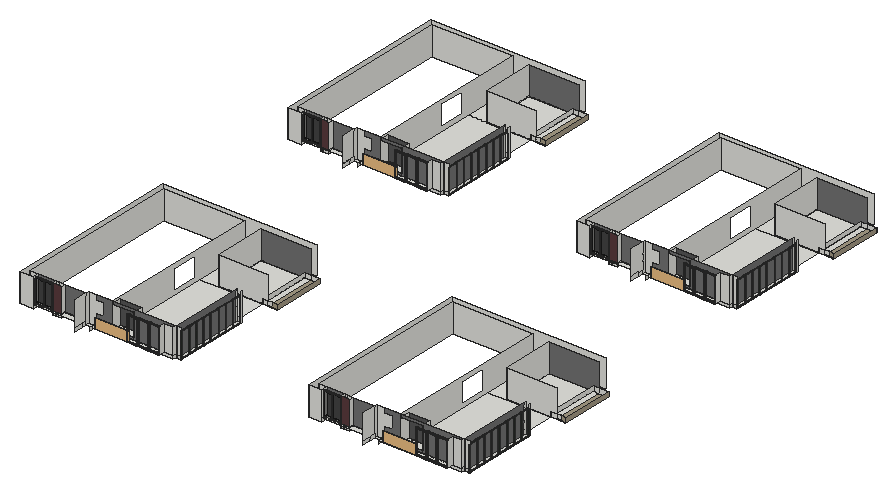
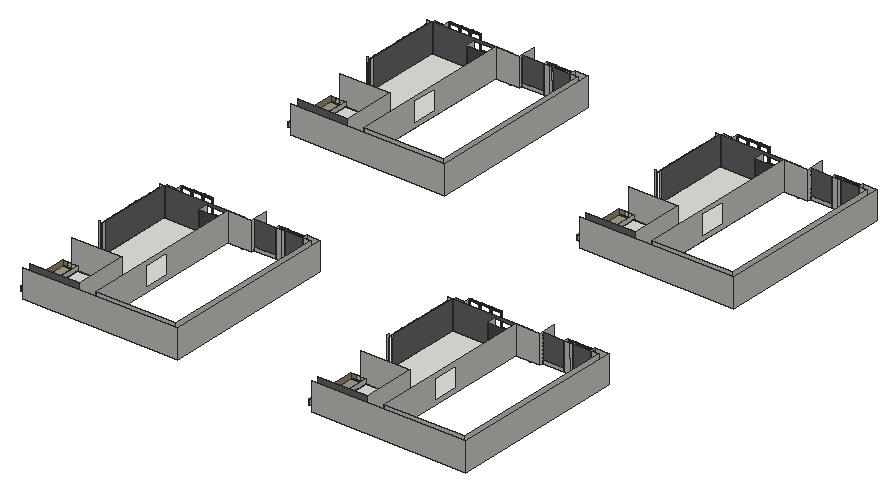
# SketchUp Ruby script. Lengths in inches.
U = 1.inch
M = Sketchup.active_model
def pt(a) = Geom::Point3d.new(a.map { |v| v * U })
def face(e, loops, mat)
  f = e.add_face(loops[0].map { |a| pt(a) })
  loops[1..].each { |l| e.add_face(l.map { |a| pt(a) }).erase! }
  f.material = f.back_material = mat if mat
  f
end
# faces: each face lists its corners as indices into pts; further lists are holes
def faces(e, pts, list, mat = nil) = list.each { |f| face(e, (f[0].is_a?(Array) ? f : [f]).map { |l| l.map { |i| pts[i] } }, mat) }
# xy, xz, yz: faces in a plane at the given z, y or x. An outline is a flat list of corners, or four numbers for a rectangle; further outlines are holes
def ring(l) = l.size == 4 ? [[l[0], l[1]], [l[2], l[1]], [l[2], l[3]], [l[0], l[3]]] : l.each_slice(2).to_a
def flat(e, list, mat, &to3) = list.each { |f| face(e, (f[0].is_a?(Array) ? f : [f]).map { |l| ring(l).map { |u, v| to3.(u, v) } }, mat) }
def xy(e, z, list, mat = nil) = flat(e, list, mat) { |x, y| [x, y, z] }
def xz(e, y, list, mat = nil) = flat(e, list, mat) { |x, z| [x, y, z] }
def yz(e, x, list, mat = nil) = flat(e, list, mat) { |y, z| [x, y, z] }
def lines(e, pts, list) = list.each { |a, b| e.add_line(pt(pts[a]), pt(pts[b])) }
# prism: a flat outline (further loops are holes) pulled along v
def prism(e, loops, v, mat = nil)
  f = face(e, loops, mat); d = Geom::Vector3d.new(v.map { |x| x * U })
  f.pushpull(f.normal.samedirection?(d) ? d.length : -d.length)
end
def box(e, o, s, mat = nil) = prism(e, [[o, [o[0] + s[0], o[1], o[2]], [o[0] + s[0], o[1] + s[1], o[2]], [o[0], o[1] + s[1], o[2]]]], [0, 0, s[2]], mat)
def at(x, y, z, deg = 0) = Geom::Transformation.translation(pt([x, y, z])) * Geom::Transformation.rotation(ORIGIN, Z_AXIS, deg.degrees)
def axes(o, x, y, z) = Geom::Transformation.new([*x, 0, *y, 0, *z, 0, *pt(o).to_a, 1])
def part(name) = M.definitions.add(name)
# library, detail: a bought-in or finely detailed component or shape, given as its bounding box
def library(name, o, s) = part(name).tap { |d| box(d.entities, o, s) }
def detail(e, o, s) = box(e.add_group.entities, o, s)
def put(e, d, t, mat = nil) = e.add_instance(d, t).tap { |i| i.material = mat if mat }
def group(e, t, mat = nil) = e.add_group.tap { |g| g.transformation = t; g.material = mat if mat }.entities
root = M.entities
M.materials.add("Glass_Tinted_Gray").color = [0, 0, 0]
M.materials["Glass_Tinted_Gray"].alpha = 0.125
M.materials.add("Glazing").color = [128, 128, 128]
M.materials["Glazing"].alpha = 0.05
M.materials.add("Powdercoating").color = [41, 44, 40]
M.materials.add("Wine2").color = [0, 0, 0]
M.materials["Wine2"].alpha = 0
M.materials.add("[0130_Gainsboro]").color = [39, 45, 50]
M.materials.add("[0135_DarkGray]").color = [81, 81, 81]
M.materials.add("[Color M05]").color = [114, 114, 114]
M.materials.add("[Color M06]").color = [86, 86, 86]
M.materials.add("[Concrete Tile]").color = [165, 155, 133]
M.materials.add("[Granite Brown]").color = [89, 59, 61]
M.materials.add("[Mirror 02]").color = [229, 229, 229]
M.materials.add("[Terrazzo Light Blue]").color = [196, 214, 227]
c1 = part("Group\#15")
xy(c1.entities,0,[[0,-55.94,0.71,45.94]])
xy(c1.entities,0.2,[[0,-55.94,0.47,45.94],[0.47,45.94,0.71,46.42]])
xy(c1.entities,2.36,[[0.47,-55.94,0.71,46.42]])
xz(c1.entities,-55.94,[[0,0,0.71,0,0.71,2.36,0.47,2.36,0.47,0.2,0,0.2]])
xz(c1.entities,45.94,[[0,0,0.71,0.2]])
xz(c1.entities,46.42,[[0.47,0.2,0.71,2.36]])
yz(c1.entities,0,[[-55.94,0,45.94,0.2]])
yz(c1.entities,0.47,[[-55.94,0.2,46.42,2.36]])
yz(c1.entities,0.71,[[-55.94,0,45.94,0,45.94,0.2,46.42,0.2,46.42,2.36,-55.94,2.36]])
c2 = part("Group\#7")
xy(c2.entities,0,[[0,-59.09,0.71,45.94]])
xy(c2.entities,0.2,[[0,-59.09,0.47,45.94],[0.47,45.94,0.71,46.42]])
xy(c2.entities,2.36,[[0.47,-59.09,0.71,46.42]])
xz(c2.entities,-59.09,[[0,0,0.71,0,0.71,2.36,0.47,2.36,0.47,0.2,0,0.2]])
xz(c2.entities,45.94,[[0,0,0.71,0.2]])
xz(c2.entities,46.42,[[0.47,0.2,0.71,2.36]])
yz(c2.entities,0,[[-59.09,0,45.94,0.2]])
yz(c2.entities,0.47,[[-59.09,0.2,46.42,2.36]])
yz(c2.entities,0.71,[[-59.09,0,45.94,0,45.94,0.2,46.42,0.2,46.42,2.36,-59.09,2.36]])
c3 = part("Group\#16")
prism(c3.entities,[[[0.47,-56.18,0.2],[0,-56.18,0.2],[0,-56.18,0],[0.71,-56.18,0],[0.71,-56.18,2.36],[0.47,-56.18,2.36]]],[0,28.68,0])
c4 = part("Group\#10")
box(c4.entities,[-0.73,0,0],[27.99,0.55,102.05])
c5 = part("Group\#18")
xy(c5.entities,0,[[0.47,-56.18,0.47,-55.47,0,-55.47,0,-28.21,1.18,-28.21,1.18,-56.18]])
xy(c5.entities,0.2,[[0.71,-56.18,1.18,-28.21],[0,-55.47,0.47,-28.21],[0.47,-28.21,0.71,-27.74]])
xy(c5.entities,2.36,[[0.47,-56.18,0.71,-27.74]])
xz(c5.entities,-56.18,[[0.47,0,1.18,0,1.18,0.2,0.71,0.2,0.71,2.36,0.47,2.36]])
xz(c5.entities,-55.47,[[0,0,0.47,0.2]])
xz(c5.entities,-28.21,[[0,0,1.18,0.2]])
xz(c5.entities,-27.74,[[0.47,0.2,0.71,2.36]])
yz(c5.entities,0,[[-55.47,0,-28.21,0.2]])
yz(c5.entities,0.47,[[-56.18,0,-55.47,0.2],[-56.18,0.2,-27.74,2.36]])
yz(c5.entities,0.71,[[-56.18,0.2,-27.74,2.36]])
yz(c5.entities,1.18,[[-56.18,0,-28.21,0.2]])
c6 = part("Group\#34")
xy(c6.entities,0,[[-20.45,0,7.76,1.22]])
xy(c6.entities,0.06,[[-20.39,0.06,7.7,1.22]])
xy(c6.entities,0.47,[[-19.98,0,7.28,0.06]])
xy(c6.entities,101.89,[[-19.98,0,7.28,0.06]])
xy(c6.entities,102.3,[[-20.39,0.06,7.7,1.22]])
xy(c6.entities,102.36,[[-20.45,0,7.76,1.22]])
xz(c6.entities,0,[[[-20.45,0,7.76,102.36],[-19.98,0.47,7.28,101.89]]])
xz(c6.entities,0.06,[[[-20.39,0.06,7.7,102.3],[-19.98,0.47,7.28,101.89]]])
xz(c6.entities,1.22,[[[-20.45,0,7.76,102.36],[-20.39,0.06,7.7,102.3]]])
yz(c6.entities,-20.45,[[0,0,1.22,102.36]])
yz(c6.entities,-20.39,[[0.06,0.06,1.22,102.3]])
yz(c6.entities,-19.98,[[0,0.47,0.06,101.89]])
yz(c6.entities,7.28,[[0,0.47,0.06,101.89]])
yz(c6.entities,7.7,[[0.06,0.06,1.22,102.3]])
yz(c6.entities,7.76,[[0,0,1.22,102.36]])
c7 = part("Group\#6")
put(c7.entities,c1,axes([27.97,0,7.875],[1,0,0],[0,0,-1],[0,1,0]),"Powdercoating")
put(c7.entities,c2,axes([0.71,0,6.8],[-1,0,0],[0,0,-0.97687],[0,1,0]),"Powdercoating")
put(c7.entities,c3,axes([-27.5,0,-38.07],[0,0,-1],[-1,0,0],[0,1,0]),"Powdercoating")
put(c7.entities,c4,at(1.12,0.35,-38.39),"Glazing")
put(c7.entities,c5,axes([-27.5,0,63.35],[0,0,1],[-1,0,0],[0,1,0]),"Powdercoating")
put(c7.entities,c6,at(20.6875,1.0625,-38.54),"Powdercoating")
c8 = part("Sliding door assembly")
put(c8.entities,c7,at(-1.18,4.5,38.86))
g1 = group(c8.entities,at(84.74,4.5,38.86))
put(g1,c1,axes([-27.97,0,7.875],[-1,0,0],[0,0,-1],[0,1,0]),"Powdercoating")
put(g1,c2,axes([-0.71,0,6.8],[1,0,0],[0,0,-0.97687],[0,1,0]),"Powdercoating")
put(g1,c3,axes([27.5,0,-38.07],[0,0,-1],[1,0,0],[0,1,0]),"Powdercoating")
put(g1,c4,axes([-1.12,0.35,-38.39],[-1,0,0],[0,1,0],[0,0,1]),"Glazing")
put(g1,c5,axes([27.5,0,63.35],[0,0,1],[1,0,0],[0,1,0]),"Powdercoating")
put(g1,c6,axes([-20.6875,1.0625,-38.54],[-1,0,0],[0,1,0],[0,0,1]),"Powdercoating")
g2 = group(c8.entities,at(56.0625,4.5,38.86))
put(g2,c1,axes([-27.97,0,7.875],[-1,0,0],[0,0,-1],[0,1,0]),"Powdercoating")
put(g2,c3,axes([27.5,0,-38.07],[0,0,-1],[1,0,0],[0,1,0]),"Powdercoating")
put(g2,c4,axes([-1.12,0.35,-38.39],[-1,0,0],[0,1,0],[0,0,1]),"Glazing")
put(g2,c5,axes([27.5,0,63.35],[0,0,1],[1,0,0],[0,1,0]),"Powdercoating")
put(g2,c6,axes([-20.6875,1.0625,-38.54],[-1,0,0],[0,1,0],[0,0,1]),"Powdercoating")
g3 = group(g2,at(-0.71,0,6.8),"Powdercoating")
xy(g3,-45.34,[[0.47,0.2,0.71,2.36]])
xy(g3,-44.88,[[0,0,0.71,0.2]])
xy(g3,57.73,[[0,0,0.71,0,0.71,2.36,0.47,2.36,0.47,0.2,0,0.2]])
xz(g3,0,[[0,-44.88,0.71,57.73]])
xz(g3,0.2,[[0.47,-45.34,0.71,-44.88],[0,-44.88,0.47,57.73]])
xz(g3,2.36,[[0.47,-45.34,0.71,57.73]])
yz(g3,0,[[0,-44.88,0.2,57.73]])
yz(g3,0.47,[[0.2,-45.34,2.36,57.73]])
yz(g3,0.71,[[0.2,-45.34,2.36,-45.34,2.36,57.73,0,57.73,0,-44.88,0.2,-44.88]])
put(c8.entities,c7,axes([-33.94,4.5,38.86],[1.14218,0,0],[0,1,0],[0,0,1]))
c9 = part("sliding door")
put(c9.entities,c8,at(0,-4.5,-0.08))
c10 = part("Framed glazing panel")
xy(c10.entities,0,[[0,-0.98,43.07,0],[0,0,43.07,1.4]],"[0130_Gainsboro]")
xy(c10.entities,0.3,[[0.3,-1.43,42.77,-0.98]],"[0130_Gainsboro]")
xy(c10.entities,2.95,[[2.95,-1.43,40.12,-0.63],[2.95,-0.63,40.12,0],[2.95,0,40.12,0.64],[2.95,0.64,40.12,1.4]],"[0130_Gainsboro]")
xy(c10.entities,3.54,[[3.54,-0.63,39.53,0],[3.54,0,39.53,0.64]],"[0130_Gainsboro]")
xy(c10.entities,111.8125,[[3.54,-0.63,39.53,0],[3.54,0,39.53,0.64]],"[0130_Gainsboro]")
xy(c10.entities,112.4,[[2.95,-1.43,40.12,-0.63],[2.95,-0.63,40.12,0],[2.95,0,40.12,0.64],[2.95,0.64,40.12,1.4]],"[0130_Gainsboro]")
xy(c10.entities,115.05,[[0.3,-1.43,42.77,-0.98]],"[0130_Gainsboro]")
xy(c10.entities,115.35,[[0,-0.98,43.07,0],[0,0,43.07,1.4]],"[0130_Gainsboro]")
xz(c10.entities,-1.43,[[[0.3,0.3,42.77,115.05],[2.95,2.95,40.12,112.4]]],"[0130_Gainsboro]")
xz(c10.entities,-0.98,[[[0,0,43.07,115.35],[0.3,0.3,42.77,115.05]]],"[0130_Gainsboro]")
xz(c10.entities,-0.63,[[[2.95,2.95,40.12,112.4],[3.54,3.54,39.53,111.8125]]],"[0130_Gainsboro]")
xz(c10.entities,0,[[3.54,3.54,39.53,111.8125]],"Wine2")
xz(c10.entities,0,[[[0,0,43.07,115.35],[2.95,2.95,40.12,112.4]],[[2.95,2.95,40.12,112.4],[3.54,3.54,39.53,111.8125]]],"[0130_Gainsboro]")
xz(c10.entities,0.64,[[[2.95,2.95,40.12,112.4],[3.54,3.54,39.53,111.8125]]],"[0130_Gainsboro]")
xz(c10.entities,1.4,[[[0,0,43.07,115.35],[2.95,2.95,40.12,112.4]]],"[0130_Gainsboro]")
yz(c10.entities,0,[[-0.98,0,0,115.35],[0,0,1.4,115.35]],"[0130_Gainsboro]")
yz(c10.entities,0.3,[[-1.43,0.3,-0.98,115.05]],"[0130_Gainsboro]")
yz(c10.entities,2.95,[[-1.43,2.95,-0.63,112.4],[-0.63,2.95,0,112.4],[0,2.95,0.64,112.4],[0.64,2.95,1.4,112.4]],"[0130_Gainsboro]")
yz(c10.entities,3.54,[[-0.63,3.54,0,111.8125],[0,3.54,0.64,111.8125]],"[0130_Gainsboro]")
yz(c10.entities,39.53,[[-0.63,3.54,0,111.8125],[0,3.54,0.64,111.8125]],"[0130_Gainsboro]")
yz(c10.entities,40.12,[[-1.43,2.95,-0.63,112.4],[-0.63,2.95,0,112.4],[0,2.95,0.64,112.4],[0.64,2.95,1.4,112.4]],"[0130_Gainsboro]")
yz(c10.entities,42.77,[[-1.43,0.3,-0.98,115.05]],"[0130_Gainsboro]")
yz(c10.entities,43.07,[[-0.98,0,0,115.35],[0,0,1.4,115.35]],"[0130_Gainsboro]")
c11 = part("Glazed panel assembly")
put(c11.entities,c10,axes([90.57,1.43,0],[1.05148,0,0],[0,1,0],[0,0,1]))
put(c11.entities,c10,axes([0,1.43,0],[1.05148,0,0],[0,1,0],[0,0,1]))
put(c11.entities,c10,axes([45.29,1.43,0],[1.05148,0,0],[0,1,0],[0,0,1]))
c12 = part("PENTEK_RP Fineline 50S_Sliding_DoorCase_E1")
box(c12.entities,[0,0,0],[1.51,3.66,99.27],"[0135_DarkGray]")
c13 = part("PENTEK_RP Fineline 50S_SlidingDooe_Case_E2")
box(c13.entities,[0,0,0],[96.25,3.66,1.51],"[0135_DarkGray]")
c14 = part("pentek_RP Fineline 50S_SlidingDoor_Case")
put(c14.entities,c12,at(97.76,0,0))
put(c14.entities,c13,at(1.51,0,0))
put(c14.entities,c12,at(0,0,0))
put(c14.entities,c13,at(1.51,0,97.76))
c15 = part("PENTEK_RP Fineline 50S_SlidingDoor_GlazingBead_2")
box(c15.entities,[0,0,0],[0.56,0.59,94.39],"[0135_DarkGray]")
c16 = part("PENTEK_RP Fineline 50S_SlidingDoor_Glass")
box(c16.entities,[0,0,0],[46.58,0.16,94.39],"Glass_Tinted_Gray")
c17 = part("PENTEK_RP Fineline 50S_SlidingDoor_GlazingBead")
box(c17.entities,[0,0,0],[45.47,0.59,0.56],"[0135_DarkGray]")
c18 = part("PENTEK_RP Fineline 50S_SlidingDoor_Leaf_E1")
xy(c18.entities,0,[[0,0,0.93,1.97],[0.93,1.57,1.49,1.97]],"[0135_DarkGray]")
xy(c18.entities,96.25,[[0,0,0.93,0,0.93,1.57,1.49,1.57,1.49,1.97,0,1.97]],"[0135_DarkGray]")
xz(c18.entities,0,[[0,0,0.93,96.25]],"[0135_DarkGray]")
xz(c18.entities,1.57,[[0.93,0,1.49,95.32],[0.93,95.32,1.49,96.25]],"[0135_DarkGray]")
xz(c18.entities,1.97,[[0,0,1.49,96.25]],"[0135_DarkGray]")
yz(c18.entities,0,[[0,0,1.97,96.25]],"[0135_DarkGray]")
yz(c18.entities,0.93,[[0,0,1.57,0.93],[0,0.93,1.57,95.32],[0,95.32,1.57,96.25]],"[0135_DarkGray]")
yz(c18.entities,1.49,[[1.57,0,1.97,95.32],[1.57,95.32,1.97,96.25]],"[0135_DarkGray]")
c19 = part("PENTEK_RP Fineline 50S_SlidingDoor_Leaf_E2")
xy(c19.entities,0,[[0,0,0,1.57,0.56,1.57,0.56,1.97,46.02,1.97,46.02,1.57,46.58,1.57,46.58,0]],"[0135_DarkGray]")
xy(c19.entities,0.93,[[0,0,46.58,1.57]],"[0135_DarkGray]")
xy(c19.entities,1.49,[[0.56,1.57,46.02,1.97]],"[0135_DarkGray]")
xz(c19.entities,0,[[0,0,46.58,0.93]],"[0135_DarkGray]")
xz(c19.entities,1.57,[[0,0,0.56,0.93],[46.02,0,46.58,0.93],[0.56,0.93,46.02,1.49]],"[0135_DarkGray]")
xz(c19.entities,1.97,[[0.56,0,46.02,1.49]],"[0135_DarkGray]")
yz(c19.entities,0,[[0,0,1.57,0.93]],"[0135_DarkGray]")
yz(c19.entities,0.56,[[1.57,0,1.97,0.93],[1.57,0.93,1.97,1.49]],"[0135_DarkGray]")
yz(c19.entities,46.02,[[1.57,0,1.97,0.93],[1.57,0.93,1.97,1.49]],"[0135_DarkGray]")
yz(c19.entities,46.58,[[0,0,1.57,0.93]],"[0135_DarkGray]")
c20 = part("PENTEK_RP Fineline S_SlidingDoor_Leaf1")
put(c20.entities,c15,at(0.93,0,0.93))
put(c20.entities,c15,at(46.96,0,0.93))
put(c20.entities,c16,at(1.49,1.42,0.93))
put(c20.entities,c17,at(1.49,0,0.93))
put(c20.entities,c16,at(1.49,0.59,0.93),"[Terrazzo Light Blue]")
put(c20.entities,c18,at(0,0,0))
put(c20.entities,c18,axes([48.44,0,0],[-1,0,0],[0,1,0],[0,0,1]))
put(c20.entities,c19,axes([0.93,0,96.25],[1,0,0],[0,1,0],[0,0,-1]))
put(c20.entities,c19,at(0.93,0,0))
put(c20.entities,c17,at(1.49,0,94.77))
c21 = part("PENTEK_RP Fineline 50S_SlidingDoor_Leaf2")
put(c21.entities,c16,at(1.49,1.42,0.93))
put(c21.entities,c17,at(1.49,0,94.77))
put(c21.entities,c15,at(46.96,0,0.93))
put(c21.entities,c16,at(1.49,0.59,0.93),"[Mirror 02]")
put(c21.entities,c15,at(0.93,0,0.93))
put(c21.entities,c18,at(0,0,0))
put(c21.entities,c18,axes([48.44,0,0],[-1,0,0],[0,1,0],[0,0,1]))
put(c21.entities,c17,at(1.49,0,0.93))
put(c21.entities,c19,axes([0.93,0,96.25],[1,0,0],[0,1,0],[0,0,-1]))
put(c21.entities,c19,at(0.93,0,0))
c22 = part("PENTEK - Slimmest Steel Sliding Door / Window\#1")
put(c22.entities,c14,at(0,-1.88,-0.09))
put(c22.entities,c20,at(1.51,-2.27,1.42))
put(c22.entities,c21,at(49.32,-0.3,1.42))
c23 = library("Glass Railing",[0,0,0],[139.5,4.76,42])
xy(root,1392,[[523.04,1822.9375,523.04,1836.125,557.4,1836.125,557.4,1835.1875,557.88,1835.1875,557.88,1822.9375],[557.88,1822.9375,625.125,1835.1875],[625.125,1822.9375,890.875,1835.1875],[1741.23,1822.9375,1741.23,1836.125,1775.59,1836.125,1775.59,1835.1875,1776.07,1835.1875,1776.07,1822.9375],[1776.07,1822.9375,1843.3125,1835.1875],
  [1843.3125,1822.9375,2109.0625,1835.1875],[557.4,1835.1875,625.125,1836.125],[625.125,1835.1875,890.875,2295.875],[894.3125,1835.1875,913.875,2156.01],[1775.59,1835.1875,1843.3125,1836.125],
  [1843.3125,1835.1875,2109.0625,2295.875],[2112.5,1835.1875,2132.0625,2156.01],[625.125,2295.875,704.25,2518.89],[704.25,2295.875,890.875,2518.89],[890.875,2295.875,913.875,2518.89],
  [1843.3125,2295.875,1922.4375,2518.89],[1922.4375,2295.875,2109.0625,2518.89],[2109.0625,2295.875,2132.0625,2518.89],[625.125,2518.89,890.875,2531.375],[1843.3125,2518.89,2109.0625,2531.375],
  [523.04,3237.625,523.04,3250.8125,557.4,3250.8125,557.4,3249.875,557.88,3249.875,557.88,3237.625],[557.88,3237.625,625.125,3249.875],[625.125,3237.625,890.875,3249.875],[1741.23,3237.625,1741.23,3250.8125,1775.59,3250.8125,1775.59,3249.875,1776.07,3249.875,1776.07,3237.625],[1776.07,3237.625,1843.3125,3249.875],
  [1843.3125,3237.625,2109.0625,3249.875],[557.4,3249.875,625.125,3250.8125],[625.125,3249.875,890.875,3710.5625],[894.3125,3249.875,913.875,3570.7],[1775.59,3249.875,1843.3125,3250.8125],
  [1843.3125,3249.875,2109.0625,3710.5625],[2112.5,3249.875,2132.0625,3570.7],[625.125,3710.5625,704.25,3933.57],[704.25,3710.5625,890.875,3933.57],[890.875,3710.5625,913.875,3933.57],
  [1843.3125,3710.5625,1922.4375,3933.57],[1922.4375,3710.5625,2109.0625,3933.57],[2109.0625,3710.5625,2132.0625,3933.57],[625.125,3933.57,890.875,3946.0625],[1843.3125,3933.57,2109.0625,3946.0625]])
xy(root,1392,[[913.875,2295.875,954.6875,2518.89],[2132.0625,2295.875,2172.875,2518.89],[913.875,3710.5625,954.6875,3933.57],[2132.0625,3710.5625,2172.875,3933.57]],"[Concrete Tile]")
xy(root,1393.75,[[704.25,2295.875,890.875,2518.89],[1922.4375,2295.875,2109.0625,2518.89],[704.25,3710.5625,890.875,3933.57],[1922.4375,3710.5625,2109.0625,3933.57]])
xy(root,1404.2,[[646.53,1835.1875,662.84,1873.375],[662.84,1835.1875,664.52,1873.375],[664.52,1835.1875,715.63,1873.375],[1864.72,1835.1875,1881.02,1873.375],[1881.02,1835.1875,1882.71,1873.375],
  [1882.71,1835.1875,1933.82,1873.375],[646.53,3249.875,662.84,3288.0625],[662.84,3249.875,664.52,3288.0625],[664.52,3249.875,715.63,3288.0625],[1864.72,3249.875,1881.02,3288.0625],
  [1881.02,3249.875,1882.71,3288.0625],[1882.71,3249.875,1933.82,3288.0625]])
xy(root,1404.51,[[625.7,1835.1875,646.53,1873.375],[1843.88,1835.1875,1864.72,1873.375],[625.7,3249.875,646.53,3288.0625],[1843.88,3249.875,1864.72,3288.0625]])
xy(root,1404.6875,[[557.88,1799.9375,851.78,1822.9375],[1776.07,1799.9375,2069.97,1822.9375],[557.88,3214.625,851.78,3237.625],[1776.07,3214.625,2069.97,3237.625]])
xy(root,1404.6875,[[557.4,1799.9375,557.88,1822.9375],[1775.59,1799.9375,1776.07,1822.9375],[557.4,3214.625,557.88,3237.625],[1775.59,3214.625,1776.07,3237.625]],"[Granite Brown]")
xy(root,1407.4375,[[319.53,1799.9375,523.04,1799.9375,523.04,1822.9375,431.33,1822.9375,431.33,1806.5625,405.58,1806.5625,405.58,1822.9375,319.53,1822.9375],[1537.72,1799.9375,1741.23,1799.9375,1741.23,1822.9375,1649.52,1822.9375,1649.52,1806.5625,1623.77,1806.5625,1623.77,1822.9375,1537.72,1822.9375],[319.53,3214.625,523.04,3214.625,523.04,3237.625,431.33,3237.625,431.33,3221.25,405.58,3221.25,405.58,3237.625,319.53,3237.625],[1537.72,3214.625,1741.23,3214.625,1741.23,3237.625,1649.52,3237.625,1649.52,3221.25,1623.77,3221.25,1623.77,3237.625,1537.72,3237.625]])
xz(root,1799.9375,[[262.875,1392,319.53,1512],[1481.0625,1392,1537.72,1512]])
xz(root,1799.9375,[[557.4,1392,557.88,1404.6875],[1775.59,1392,1776.07,1404.6875]],"[Granite Brown]")
xz(root,1806.5625,[[405.58,1392,405.58,1407.4375,394.85,1407.49,394.77,1392.05],[405.58,1392,405.66,1407.4375,405.58,1407.4375],[405.58,1392,431.33,1392,431.33,1407.4375,405.66,1407.4375],[1623.77,1392,1623.77,1407.4375,1613.04,1407.49,1612.96,1392.05],[1623.77,1392,1623.85,1407.4375,1623.77,1407.4375],
  [1623.77,1392,1649.52,1392,1649.52,1407.4375,1623.85,1407.4375]])
xz(root,1806.5625,[[405.58,1407.4375,431.33,1407.4375,431.33,1512,406.18,1512,395.37,1512.05,394.85,1407.49],[1623.77,1407.4375,1649.52,1407.4375,1649.52,1512,1624.37,1512,1613.56,1512.05,1613.04,1407.49]],"[Granite Brown]")
xz(root,1822.9375,[[285.875,1392,319.53,1512],[319.53,1392,405.58,1392,394.77,1392.05,394.85,1407.4375,319.53,1407.4375],[405.58,1392,394.77,1392.05,394.85,1407.4375,405.58,1407.4375],[405.58,1392,406.18,1512,395.37,1512,394.85,1407.4375,405.58,1407.4375],[405.58,1392,406.18,1512,431.33,1512,431.33,1392],
  [431.33,1392,523.04,1407.4375],[557.88,1392,625.125,1404.6875],[625.125,1392,890.875,1404.6875],[1504.0625,1392,1537.72,1512],[1537.72,1392,1623.77,1392,1612.96,1392.05,1613.03,1407.4375,1537.72,1407.4375],
  [1623.77,1392,1612.96,1392.05,1613.03,1407.4375,1623.77,1407.4375],[1623.77,1392,1624.37,1512,1613.56,1512,1613.03,1407.4375,1623.77,1407.4375],[1623.77,1392,1624.37,1512,1649.52,1512,1649.52,1392],[1649.52,1392,1741.23,1407.4375],[1776.07,1392,1843.3125,1404.6875],
  [1843.3125,1392,2109.0625,1404.6875],[851.78,1404.6875,890.875,1512],[2069.97,1404.6875,2109.0625,1512]])
xz(root,1822.9375,[[319.53,1407.4375,394.85,1407.4375,395.37,1512,319.53,1512],[431.33,1407.4375,523.04,1512],[1537.72,1407.4375,1613.03,1407.4375,1613.56,1512,1537.72,1512],[1649.52,1407.4375,1741.23,1512]],"[Color M05]")
xz(root,1822.9375,[[557.4,1392,557.88,1404.6875],[1775.59,1392,1776.07,1404.6875]],"[Granite Brown]")
xz(root,1835.1875,[[890.875,1392,894.3125,1404.6875],[894.3125,1392,913.875,1404.6875],[2109.0625,1392,2112.5,1404.6875],[2112.5,1392,2132.0625,1404.6875],[894.3125,1404.6875,913.875,1512],
  [2112.5,1404.6875,2132.0625,1512]])
xz(root,1835.1875,[[[557.88,1392,890.875,1392,890.875,1512,557.88,1512,557.88,1494.26,588.66,1494.26,588.66,1441.98,557.88,1441.98],[646.53,1404.2,646.53,1404.51,625.7,1404.51,625.7,1502.33,715.63,1502.33,715.63,1404.2]],[[1776.07,1392,2109.0625,1392,2109.0625,1512,1776.07,1512,1776.07,1494.26,1806.84,1494.26,1806.84,1441.98,1776.07,1441.98],[1864.72,1404.2,1864.72,1404.51,1843.88,1404.51,1843.88,1502.33,1933.82,1502.33,1933.82,1404.2]]],"[Color M05]")
xz(root,1836.125,[[523.04,1392,625.125,1512],[1741.23,1392,1843.3125,1512]])
xz(root,1873.375,[[646.53,1404.2,715.63,1404.2,715.63,1502.33,625.7,1502.33,625.7,1404.51,646.53,1404.51],[1864.72,1404.2,1933.82,1404.2,1933.82,1502.33,1843.88,1502.33,1843.88,1404.51,1864.72,1404.51]],"[Color M06]")
xz(root,2156.01,[[894.3125,1392,913.875,1409.36],[2112.5,1392,2132.0625,1409.36]])
xz(root,2295.875,[[704.25,1392,890.875,1393.75],[890.875,1392,913.875,1412.8125],[913.875,1392,930.75,1393.75],[930.75,1392,954.6875,1393.75],[1922.4375,1392,2109.0625,1393.75],
  [2109.0625,1392,2132.0625,1412.8125],[2132.0625,1392,2148.9375,1393.75],[2148.9375,1392,2172.875,1393.75],[704.25,1393.75,704.25,1512,913.875,1512,913.875,1412.8125,890.875,1412.8125,890.875,1393.75],[913.875,1393.75,930.75,1412.8125],
  [1922.4375,1393.75,1922.4375,1512,2132.0625,1512,2132.0625,1412.8125,2109.0625,1412.8125,2109.0625,1393.75],[2132.0625,1393.75,2148.9375,1412.8125]])
xz(root,2295.875,[[930.75,1393.75,954.6875,1412.8125],[2148.9375,1393.75,2172.875,1412.8125]],"[Concrete Tile]")
xz(root,2518.89,[[704.25,1392,890.875,1393.75],[890.875,1392,913.875,1412.8125],[913.875,1392,954.6875,1412.8125],[1922.4375,1392,2109.0625,1393.75],[2109.0625,1392,2132.0625,1412.8125],
  [2132.0625,1392,2172.875,1412.8125]])
xz(root,2518.89,[[704.25,1393.75,890.875,1393.75,890.875,1412.8125,913.875,1412.8125,913.875,1512,704.25,1512],[1922.4375,1393.75,2109.0625,1393.75,2109.0625,1412.8125,2132.0625,1412.8125,2132.0625,1512,1922.4375,1512]],"[Color M05]")
xz(root,2531.375,[[285.875,1392,625.125,1512],[1504.0625,1392,1843.3125,1512]])
xz(root,2554.375,[[262.875,1392,913.875,1512],[1481.0625,1392,2132.0625,1512]])
xz(root,3214.625,[[262.875,1392,319.53,1512],[1481.0625,1392,1537.72,1512]])
xz(root,3214.625,[[557.4,1392,557.88,1404.6875],[1775.59,1392,1776.07,1404.6875]],"[Granite Brown]")
xz(root,3221.25,[[405.58,1392,405.58,1407.4375,394.85,1407.49,394.77,1392.05],[405.58,1392,405.66,1407.4375,405.58,1407.4375],[405.58,1392,431.33,1392,431.33,1407.4375,405.66,1407.4375],[1623.77,1392,1623.77,1407.4375,1613.04,1407.49,1612.96,1392.05],[1623.77,1392,1623.85,1407.4375,1623.77,1407.4375],
  [1623.77,1392,1649.52,1392,1649.52,1407.4375,1623.85,1407.4375]])
xz(root,3221.25,[[405.58,1407.4375,431.33,1407.4375,431.33,1512,406.18,1512,395.37,1512.05,394.85,1407.49],[1623.77,1407.4375,1649.52,1407.4375,1649.52,1512,1624.37,1512,1613.56,1512.05,1613.04,1407.49]],"[Granite Brown]")
xz(root,3237.625,[[285.875,1392,319.53,1512],[319.53,1392,405.58,1392,394.77,1392.05,394.85,1407.4375,319.53,1407.4375],[405.58,1392,394.77,1392.05,394.85,1407.4375,405.58,1407.4375],[405.58,1392,406.18,1512,395.37,1512,394.85,1407.4375,405.58,1407.4375],[405.58,1392,406.18,1512,431.33,1512,431.33,1392],
  [431.33,1392,523.04,1407.4375],[557.88,1392,625.125,1404.6875],[625.125,1392,890.875,1404.6875],[1504.0625,1392,1537.72,1512],[1537.72,1392,1623.77,1392,1612.96,1392.05,1613.03,1407.4375,1537.72,1407.4375],
  [1623.77,1392,1612.96,1392.05,1613.03,1407.4375,1623.77,1407.4375],[1623.77,1392,1624.37,1512,1613.56,1512,1613.03,1407.4375,1623.77,1407.4375],[1623.77,1392,1624.37,1512,1649.52,1512,1649.52,1392],[1649.52,1392,1741.23,1407.4375],[1776.07,1392,1843.3125,1404.6875],
  [1843.3125,1392,2109.0625,1404.6875],[851.78,1404.6875,890.875,1512],[2069.97,1404.6875,2109.0625,1512]])
xz(root,3237.625,[[319.53,1407.4375,394.85,1407.4375,395.37,1512,319.53,1512],[431.33,1407.4375,523.04,1512],[1537.72,1407.4375,1613.03,1407.4375,1613.56,1512,1537.72,1512],[1649.52,1407.4375,1741.23,1512]],"[Color M05]")
xz(root,3237.625,[[557.4,1392,557.88,1404.6875],[1775.59,1392,1776.07,1404.6875]],"[Granite Brown]")
xz(root,3249.875,[[890.875,1392,894.3125,1404.6875],[894.3125,1392,913.875,1404.6875],[2109.0625,1392,2112.5,1404.6875],[2112.5,1392,2132.0625,1404.6875],[894.3125,1404.6875,913.875,1512],
  [2112.5,1404.6875,2132.0625,1512]])
xz(root,3249.875,[[[557.88,1392,890.875,1392,890.875,1512,557.88,1512,557.88,1494.26,588.66,1494.26,588.66,1441.98,557.88,1441.98],[646.53,1404.2,646.53,1404.51,625.7,1404.51,625.7,1502.33,715.63,1502.33,715.63,1404.2]],[[1776.07,1392,2109.0625,1392,2109.0625,1512,1776.07,1512,1776.07,1494.26,1806.84,1494.26,1806.84,1441.98,1776.07,1441.98],[1864.72,1404.2,1864.72,1404.51,1843.88,1404.51,1843.88,1502.33,1933.82,1502.33,1933.82,1404.2]]],"[Color M05]")
xz(root,3250.8125,[[523.04,1392,625.125,1512],[1741.23,1392,1843.3125,1512]])
xz(root,3288.0625,[[646.53,1404.2,715.63,1404.2,715.63,1502.33,625.7,1502.33,625.7,1404.51,646.53,1404.51],[1864.72,1404.2,1933.82,1404.2,1933.82,1502.33,1843.88,1502.33,1843.88,1404.51,1864.72,1404.51]],"[Color M06]")
xz(root,3570.7,[[894.3125,1392,913.875,1409.36],[2112.5,1392,2132.0625,1409.36]])
xz(root,3710.5625,[[704.25,1392,890.875,1393.75],[890.875,1392,913.875,1412.8125],[913.875,1392,930.75,1393.75],[930.75,1392,954.6875,1393.75],[1922.4375,1392,2109.0625,1393.75],
  [2109.0625,1392,2132.0625,1412.8125],[2132.0625,1392,2148.9375,1393.75],[2148.9375,1392,2172.875,1393.75],[704.25,1393.75,704.25,1512,913.875,1512,913.875,1412.8125,890.875,1412.8125,890.875,1393.75],[913.875,1393.75,930.75,1412.8125],
  [1922.4375,1393.75,1922.4375,1512,2132.0625,1512,2132.0625,1412.8125,2109.0625,1412.8125,2109.0625,1393.75],[2132.0625,1393.75,2148.9375,1412.8125]])
xz(root,3710.5625,[[930.75,1393.75,954.6875,1412.8125],[2148.9375,1393.75,2172.875,1412.8125]],"[Concrete Tile]")
xz(root,3933.57,[[704.25,1392,890.875,1393.75],[890.875,1392,913.875,1412.8125],[913.875,1392,954.6875,1412.8125],[1922.4375,1392,2109.0625,1393.75],[2109.0625,1392,2132.0625,1412.8125],
  [2132.0625,1392,2172.875,1412.8125]])
xz(root,3933.57,[[704.25,1393.75,890.875,1393.75,890.875,1412.8125,913.875,1412.8125,913.875,1512,704.25,1512],[1922.4375,1393.75,2109.0625,1393.75,2109.0625,1412.8125,2132.0625,1412.8125,2132.0625,1512,1922.4375,1512]],"[Color M05]")
xz(root,3946.0625,[[285.875,1392,625.125,1512],[1504.0625,1392,1843.3125,1512]])
xz(root,3969.0625,[[262.875,1392,913.875,1512],[1481.0625,1392,2132.0625,1512]])
yz(root,262.875,[[1799.9375,1392,2554.375,1512],[3214.625,1392,3969.0625,1512]])
yz(root,285.875,[[1822.9375,1392,2531.375,1512],[3237.625,1392,3946.0625,1512]])
yz(root,319.53,[[1799.9375,1392,1822.9375,1407.4375],[3214.625,1392,3237.625,1407.4375],[1799.9375,1407.4375,1822.9375,1512],[3214.625,1407.4375,3237.625,1512]])
yz(root,405.58,[[1806.5625,1392,1822.9375,1407.4375],[3221.25,1392,3237.625,1407.4375]])
yz(root,431.33,[[1806.5625,1392,1822.9375,1407.4375],[3221.25,1392,3237.625,1407.4375],[1806.5625,1407.4375,1822.9375,1512],[3221.25,1407.4375,3237.625,1512]])
yz(root,523.04,[[1763.25,1392,1799.9375,1407.4375],[1799.9375,1392,1822.9375,1407.4375],[1822.9375,1392,1836.125,1512],[3177.9375,1392,3214.625,1407.4375],[3214.625,1392,3237.625,1407.4375],
  [3237.625,1392,3250.8125,1512],[1763.25,1407.4375,1822.9375,1512],[3177.9375,1407.4375,3237.625,1512]])
yz(root,557.4,[[1799.9375,1392,1822.9375,1404.6875],[3214.625,1392,3237.625,1404.6875]])
yz(root,625.125,[[[1836.125,1392,2531.375,1512],[2156.01,1409.36,2266.33,1495.04]],[[3250.8125,1392,3946.0625,1512],[3570.7,1409.36,3681.01,1495.04]]])
yz(root,625.7,[[1835.1875,1404.51,1873.375,1502.33],[3249.875,1404.51,3288.0625,1502.33]])
yz(root,646.53,[[1835.1875,1404.2,1873.375,1404.51],[3249.875,1404.2,3288.0625,1404.51]])
yz(root,704.25,[[2295.875,1392,2518.89,1393.75],[3710.5625,1392,3933.57,1393.75],[2295.875,1393.75,2518.89,1512],[3710.5625,1393.75,3933.57,1512]])
yz(root,715.63,[[1835.1875,1404.2,1873.375,1502.33],[3249.875,1404.2,3288.0625,1502.33]])
yz(root,851.78,[[1799.9375,1404.6875,1822.9375,1512],[3214.625,1404.6875,3237.625,1512]])
yz(root,890.875,[[1822.9375,1392,1835.1875,1404.6875],[2295.875,1392,2518.89,1393.75],[3237.625,1392,3249.875,1404.6875],[3710.5625,1392,3933.57,1393.75],[2295.875,1393.75,2518.89,1412.8125],
  [3710.5625,1393.75,3933.57,1412.8125],[1822.9375,1404.6875,1835.1875,1512],[3237.625,1404.6875,3249.875,1512]])
yz(root,894.3125,[[2148.83,1392,2156.01,1512],[3563.51,1392,3570.7,1512]])
yz(root,894.3125,[[1835.1875,1392,2148.83,1512],[3249.875,1392,3563.51,1512]],"[Color M05]")
yz(root,913.875,[[2148.83,1392,2156.01,1512],[3563.51,1392,3570.7,1512]])
yz(root,954.6875,[[2295.875,1392,2518.89,1412.8125],[3710.5625,1392,3933.57,1412.8125]],"[Concrete Tile]")
yz(root,1481.0625,[[1799.9375,1392,2554.375,1512],[3214.625,1392,3969.0625,1512]])
yz(root,1504.0625,[[1822.9375,1392,2531.375,1512],[3237.625,1392,3946.0625,1512]])
yz(root,1537.72,[[1799.9375,1392,1822.9375,1407.4375],[3214.625,1392,3237.625,1407.4375],[1799.9375,1407.4375,1822.9375,1512],[3214.625,1407.4375,3237.625,1512]])
yz(root,1623.77,[[1806.5625,1392,1822.9375,1407.4375],[3221.25,1392,3237.625,1407.4375]])
yz(root,1649.52,[[1806.5625,1392,1822.9375,1407.4375],[3221.25,1392,3237.625,1407.4375],[1806.5625,1407.4375,1822.9375,1512],[3221.25,1407.4375,3237.625,1512]])
yz(root,1741.23,[[1763.25,1392,1799.9375,1407.4375],[1799.9375,1392,1822.9375,1407.4375],[1822.9375,1392,1836.125,1512],[3177.9375,1392,3214.625,1407.4375],[3214.625,1392,3237.625,1407.4375],
  [3237.625,1392,3250.8125,1512],[1763.25,1407.4375,1822.9375,1512],[3177.9375,1407.4375,3237.625,1512]])
yz(root,1775.59,[[1799.9375,1392,1822.9375,1404.6875],[3214.625,1392,3237.625,1404.6875]])
yz(root,1843.3125,[[[1836.125,1392,2531.375,1512],[2156.01,1409.36,2266.33,1495.04]],[[3250.8125,1392,3946.0625,1512],[3570.7,1409.36,3681.01,1495.04]]])
yz(root,1843.88,[[1835.1875,1404.51,1873.375,1502.33],[3249.875,1404.51,3288.0625,1502.33]])
yz(root,1864.72,[[1835.1875,1404.2,1873.375,1404.51],[3249.875,1404.2,3288.0625,1404.51]])
yz(root,1922.4375,[[2295.875,1392,2518.89,1393.75],[3710.5625,1392,3933.57,1393.75],[2295.875,1393.75,2518.89,1512],[3710.5625,1393.75,3933.57,1512]])
yz(root,1933.82,[[1835.1875,1404.2,1873.375,1502.33],[3249.875,1404.2,3288.0625,1502.33]])
yz(root,2069.97,[[1799.9375,1404.6875,1822.9375,1512],[3214.625,1404.6875,3237.625,1512]])
yz(root,2109.0625,[[1822.9375,1392,1835.1875,1404.6875],[2295.875,1392,2518.89,1393.75],[3237.625,1392,3249.875,1404.6875],[3710.5625,1392,3933.57,1393.75],[2295.875,1393.75,2518.89,1412.8125],
  [3710.5625,1393.75,3933.57,1412.8125],[1822.9375,1404.6875,1835.1875,1512],[3237.625,1404.6875,3249.875,1512]])
yz(root,2112.5,[[2148.83,1392,2156.01,1512],[3563.51,1392,3570.7,1512]])
yz(root,2112.5,[[1835.1875,1392,2148.83,1512],[3249.875,1392,3563.51,1512]],"[Color M05]")
yz(root,2132.0625,[[2148.83,1392,2156.01,1512],[3563.51,1392,3570.7,1512]])
yz(root,2172.875,[[2295.875,1392,2518.89,1412.8125],[3710.5625,1392,3933.57,1412.8125]],"[Concrete Tile]")
p = [[405.58,1822.9375,1392],[405.58,1806.5625,1392],[394.77,1806.5625,1392.05],[394.77,1822.9375,1392.05],[1623.77,1822.9375,1392],[1623.77,1806.5625,1392],
  [1612.96,1806.5625,1392.05],[1612.96,1822.9375,1392.05],[405.58,3237.625,1392],[405.58,3221.25,1392],[394.77,3221.25,1392.05],[394.77,3237.625,1392.05],
  [1623.77,3237.625,1392],[1623.77,3221.25,1392],[1612.96,3221.25,1392.05],[1612.96,3237.625,1392.05],[394.85,1806.5625,1407.49],[395.37,1806.5625,1512.05],
  [395.37,1822.9375,1512.05],[395.37,1822.9375,1512],[394.85,1822.9375,1407.4375],[1613.04,1806.5625,1407.49],[1613.56,1806.5625,1512.05],[1613.56,1822.9375,1512.05],
  [1613.56,1822.9375,1512],[1613.03,1822.9375,1407.4375],[394.85,3221.25,1407.49],[395.37,3221.25,1512.05],[395.37,3237.625,1512.05],[395.37,3237.625,1512],
  [394.85,3237.625,1407.4375],[1613.04,3221.25,1407.49],[1613.56,3221.25,1512.05],[1613.56,3237.625,1512.05],[1613.56,3237.625,1512],[1613.03,3237.625,1407.4375]]
faces(root,p,[[0,1,2,3],[4,5,6,7],[8,9,10,11],[12,13,14,15],[3,2,16,17,18,19,20],[7,6,21,22,23,24,25],[11,10,26,27,28,29,30],[15,14,31,32,33,34,35]])
put(root,c9,axes([2132.0625,1879.83,1392],[0,1.302,0],[-1,0,0],[0,0,1.03877]))
put(root,c9,axes([2132.0625,2036.83,1392],[0,1.302,0],[-1,0,0],[0,0,1.03877]))
put(root,c9,axes([913.875,2036.83,1392],[0,1.302,0],[-1,0,0],[0,0,1.03877]))
put(root,c9,axes([913.875,1879.83,1392],[0,1.302,0],[-1,0,0],[0,0,1.03877]))
put(root,c9,axes([2132.0625,3294.51,1392],[0,1.302,0],[-1,0,0],[0,0,1.03877]))
put(root,c9,axes([2132.0625,3451.51,1392],[0,1.302,0],[-1,0,0],[0,0,1.03877]))
put(root,c9,axes([913.875,3451.51,1392],[0,1.302,0],[-1,0,0],[0,0,1.03877]))
put(root,c9,axes([913.875,3294.51,1392],[0,1.302,0],[-1,0,0],[0,0,1.03877]))
put(root,c11,axes([1933.82,1798.3125,1404.6875],[1,0,0],[0,1,0],[0,0,0.93029]))
put(root,c11,axes([715.63,1798.3125,1404.6875],[1,0,0],[0,1,0],[0,0,0.93029]))
put(root,c11,axes([1933.82,3213,1404.6875],[1,0,0],[0,1,0],[0,0,0.93029]))
put(root,c11,axes([715.63,3213,1404.6875],[1,0,0],[0,1,0],[0,0,0.93029]))
put(root,c22,axes([1537.72,1808.46,1405.94],[0.74394,0,0],[0,0.88,0],[0,0,1.054]))
put(root,c22,axes([319.53,1808.46,1405.94],[0.74394,0,0],[0,0.88,0],[0,0,1.054]))
put(root,c22,axes([1537.72,3223.15,1405.94],[0.74394,0,0],[0,0.88,0],[0,0,1.054]))
put(root,c22,axes([319.53,3223.15,1405.94],[0.74394,0,0],[0,0.88,0],[0,0,1.054]))
put(root,c23,at(1798.04,1796.375,1407.29))
put(root,c23,at(579.86,1796.375,1407.29))
put(root,c23,at(1798.04,3211.0625,1407.29))
put(root,c23,at(579.86,3211.0625,1407.29))
